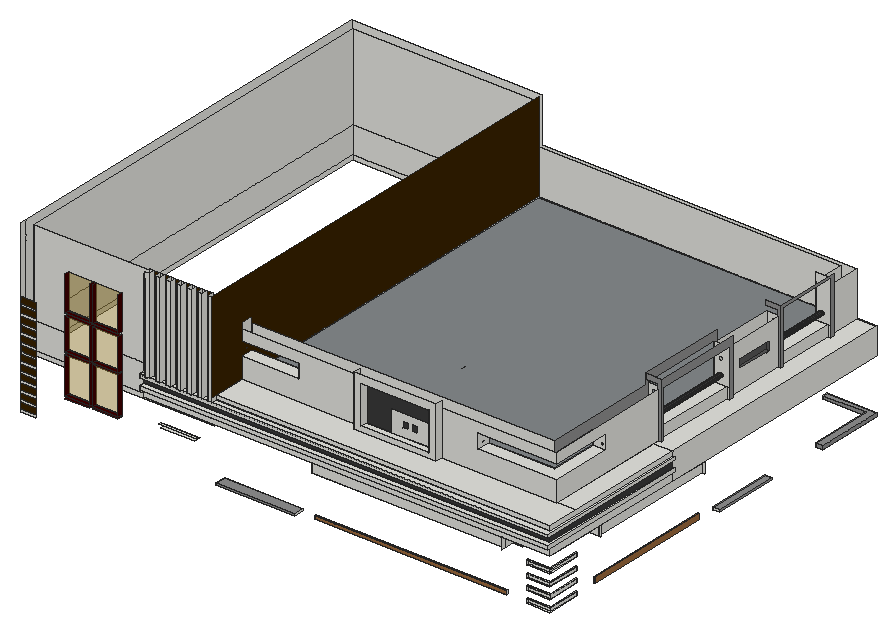
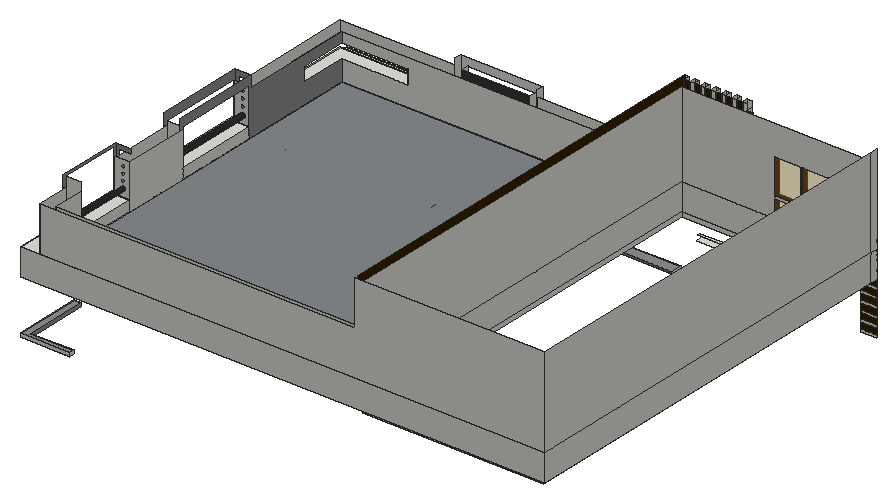
# SketchUp Ruby script. Lengths in inches.
U = 1.inch
M = Sketchup.active_model
def pt(a) = Geom::Point3d.new(a.map { |v| v * U })
def face(e, loops, mat)
  f = e.add_face(loops[0].map { |a| pt(a) })
  loops[1..].each { |l| e.add_face(l.map { |a| pt(a) }).erase! }
  f.material = f.back_material = mat if mat
  f
end
# faces: each face lists its corners as indices into pts; further lists are holes
def faces(e, pts, list, mat = nil) = list.each { |f| face(e, (f[0].is_a?(Array) ? f : [f]).map { |l| l.map { |i| pts[i] } }, mat) }
# xy, xz, yz: faces in a plane at the given z, y or x. An outline is a flat list of corners, or four numbers for a rectangle; further outlines are holes
def ring(l) = l.size == 4 ? [[l[0], l[1]], [l[2], l[1]], [l[2], l[3]], [l[0], l[3]]] : l.each_slice(2).to_a
def flat(e, list, mat, &to3) = list.each { |f| face(e, (f[0].is_a?(Array) ? f : [f]).map { |l| ring(l).map { |u, v| to3.(u, v) } }, mat) }
def xy(e, z, list, mat = nil) = flat(e, list, mat) { |x, y| [x, y, z] }
def xz(e, y, list, mat = nil) = flat(e, list, mat) { |x, z| [x, y, z] }
def yz(e, x, list, mat = nil) = flat(e, list, mat) { |y, z| [x, y, z] }
def lines(e, pts, list) = list.each { |a, b| e.add_line(pt(pts[a]), pt(pts[b])) }
# prism: a flat outline (further loops are holes) pulled along v
def prism(e, loops, v, mat = nil)
  f = face(e, loops, mat); d = Geom::Vector3d.new(v.map { |x| x * U })
  f.pushpull(f.normal.samedirection?(d) ? d.length : -d.length)
end
def box(e, o, s, mat = nil) = prism(e, [[o, [o[0] + s[0], o[1], o[2]], [o[0] + s[0], o[1] + s[1], o[2]], [o[0], o[1] + s[1], o[2]]]], [0, 0, s[2]], mat)
def at(x, y, z, deg = 0) = Geom::Transformation.translation(pt([x, y, z])) * Geom::Transformation.rotation(ORIGIN, Z_AXIS, deg.degrees)
def axes(o, x, y, z) = Geom::Transformation.new([*x, 0, *y, 0, *z, 0, *pt(o).to_a, 1])
def part(name) = M.definitions.add(name)
# library, detail: a bought-in or finely detailed component or shape, given as its bounding box
def library(name, o, s) = part(name).tap { |d| box(d.entities, o, s) }
def detail(e, o, s) = box(e.add_group.entities, o, s)
def put(e, d, t, mat = nil) = e.add_instance(d, t).tap { |i| i.material = mat if mat }
def group(e, t, mat = nil) = e.add_group.tap { |g| g.transformation = t; g.material = mat if mat }.entities
root = M.entities
M.materials.add("[Blacktop Old 01]").color = [132, 136, 139]
M.materials.add("[Color A08]").color = [56, 34, 0]
M.materials.add("[Color A08]1").color = [63, 0, 0]
M.materials.add("[Color M04]").color = [142, 142, 142]
M.materials.add("[Color M06]").color = [86, 86, 86]
M.materials.add("[Color M07]").color = [58, 58, 58]
M.materials.add("[Translucent Glass Blue]").color = [179, 149, 61]
M.materials["[Translucent Glass Blue]"].alpha = 0.5
M.materials.add("[Wood Floor]").color = [155, 105, 61]
xy(root,249,[[329.75,496.71,434.48,511.31],[455.35,504.34,712.1,506.34],[767.0625,581.49,769.0625,754.59],[767.1875,780.03,776.3125,867.13],[767.1875,951.14,767.1875,1035.15,710.3125,1035.15,710.3125,1041.15,776.3125,1041.15,776.3125,951.14]])
xy(root,249.35,[[739.88,502.4,771.75,502.4,771.75,547.34,770.25,547.34,770.25,504.84,739.88,504.84]])
xy(root,251.5625,[[329.75,496.71,434.48,511.31]],"[Color M04]")
xy(root,252.0625,[[767.1875,780.03,776.3125,867.13]],"[Color M04]")
xy(root,253.3125,[[455.35,504.34,712.1,506.34]],"[Wood Floor]")
xy(root,253.6875,[[767.1875,951.14,776.3125,951.14,776.3125,1041.15,710.3125,1041.15,710.3125,1035.15,767.1875,1035.15]],"[Color M04]")
xy(root,254.73,[[739.88,502.4,745.57,504.84],[745.57,502.4,771.75,504.84],[770.25,504.84,771.75,547.34]])
xy(root,256.0625,[[767.0625,581.49,769.0625,754.59]],"[Wood Floor]")
xy(root,264.67,[[739.88,502.4,771.75,502.4,771.75,547.34,770.25,547.34,770.25,504.77,739.88,504.77]])
xy(root,270.04,[[739.88,502.4,745.57,504.77],[745.57,502.4,771.75,504.77],[770.25,504.77,771.75,547.34]])
xy(root,279.42,[[739.88,502.4,771.75,502.4,771.75,547.34,770.0625,547.34,770.0625,504.4,739.88,504.4]])
xy(root,281.9,[[128.05,496.71,161.69,502.71],[165.04,496.71,198.99,502.71]],"[Color A08]1")
xy(root,284.79,[[739.88,502.4,745.57,504.4],[745.57,502.4,771.75,504.4],[770.0625,504.4,771.75,547.34]])
xy(root,284.92,[[128.05,496.71,161.69,502.71],[165.04,496.71,198.99,502.71]],"[Color A08]1")
xy(root,285,[[470.51,700.96,518.51,706.96]])
xy(root,286.38,[[560.85,700.96,616.42,706.96]])
xy(root,294.03,[[258.89,493.59,303.7,502.71]])
xy(root,295.73,[[739.88,502.4,745.57,504.65],[745.57,502.4,771.75,504.65],[769.8125,504.65,771.75,547.34]])
xy(root,297.5625,[[255.94,493.59,306.57,496.71]])
xy(root,301.1,[[739.88,502.4,745.57,504.65],[745.57,502.4,771.75,504.65],[769.8125,504.65,771.75,547.34]])
xy(root,306.3125,[[454.78,500.59,454.78,515.78,724.73,515.78,724.73,514.59,712.1,514.59,712.1,500.59],[758.97,581.49,758.0625,754.59,772.875,754.59,772.875,581.49]])
xy(root,321,[[329.75,496.71,329.75,700.96,710.3125,700.96,710.3125,1041.15,776.3125,1041.15,776.3125,780.03,758.0625,780.03,758.0625,754.59,758.97,581.49,758.97,566.61,724.73,566.61,724.73,515.78,455.35,515.78,455.35,516.84,434.48,516.84,434.48,496.71],[434.48,496.71,454.78,496.71,454.78,515.78,455.35,515.78,455.35,516.84,434.48,516.84],[454.78,496.71,455.35,500.59],[455.35,496.71,712.1,500.59],[712.1,496.71,724.73,514.59],
  [724.73,496.71,776.3125,502.4],[454.78,500.59,455.35,515.78],[455.35,500.59,712.1,500.59,712.1,514.59,724.73,514.59,724.73,515.78,455.35,515.78],[771.75,502.4,776.3125,566.61],[758.97,566.61,776.3125,581.49],
  [758.97,581.49,772.875,581.49,772.875,754.59,758.0625,754.59],[772.875,581.49,776.3125,700.96],[772.875,700.96,776.3125,754.59]])
xy(root,332.8125,[[233.4,489.27,776.3125,496.71],[776.3125,489.27,779.5,700.96],[329.75,496.71,776.3125,700.96]])
xy(root,334.65,[[128.05,496.71,161.69,502.71],[165.04,496.71,198.99,502.71]],"[Color A08]1")
xy(root,337.4375,[[233.4,489.27,779.5,489.27,779.5,700.96,776.3125,700.96,776.3125,496.71,233.4,496.71],[329.75,496.71,776.3125,700.96]])
xy(root,337.67,[[128.05,496.71,161.69,502.71],[165.04,496.71,198.99,502.71]],"[Color A08]1")
xy(root,347.125,[[233.4,489.27,776.3125,496.71],[776.3125,489.27,779.5,700.96],[329.75,496.71,776.3125,700.96]])
xy(root,351,[[329.75,706.96,689.4375,1035.15]])
xy(root,351.3125,[[241.19,489.02,247.4,489.27],[255.19,489.02,261.4,489.27],[269.19,489.02,275.4,489.27],[283.19,489.02,289.4,489.27],[297.19,489.02,303.4,489.27],
  [233.4,489.27,241.19,496.71],[241.19,489.27,247.4,496.71],[247.4,489.27,255.19,496.71],[255.19,489.27,261.4,496.71],[261.4,489.27,269.19,496.71],
  [269.19,489.27,275.4,496.71],[275.4,489.27,283.19,496.71],[283.19,489.27,289.4,496.71],[289.4,489.27,297.19,496.71],[297.19,489.27,303.4,496.71],
  [303.4,489.27,311.19,496.71],[311.19,489.27,317.4,496.71],[317.4,489.27,325.19,496.71],[325.19,489.27,329.75,496.71],[329.75,489.27,779.5,489.27,779.5,700.96,776.3125,700.96,776.3125,496.71,329.75,496.71]])
xy(root,357,[[329.75,496.71,776.3125,496.71,776.3125,539.27,597.14,539.27,597.14,529.59,488.01,529.59,488.01,539.27,329.75,539.27],[488.01,529.59,597.14,539.27],[329.75,539.27,750.625,539.27,750.625,700.96,733.6875,700.96,733.6875,557.27,329.75,557.27],[750.625,539.27,776.3125,700.96],[733.6875,700.96,733.6875,712.4,754.75,712.4,754.75,709.18,750.625,709.18,750.625,700.96],
  [750.625,700.96,750.625,709.18,754.75,709.18,754.75,712.4,750.625,712.4,750.625,823.78,754.75,823.78,754.75,828.03,750.625,828.03,750.625,909.39,754.75,909.39,754.75,912.34,750.625,912.34,750.625,992.73,754.75,992.73,754.75,996.8,750.625,996.8,750.625,1041.15,776.3125,1041.15,776.3125,700.96],[733.6875,823.78,733.6875,912.34,754.75,912.34,754.75,909.39,750.625,909.39,750.625,828.03,754.75,828.03,754.75,823.78]])
xy(root,357,[[329.75,557.27,733.6875,1035.15]],"[Blacktop Old 01]")
xy(root,363.72,[[496.66,529.59,587.54,539.27]])
xy(root,371.375,[[733.6875,712.4,750.625,823.78],[733.6875,912.34,750.625,992.73]])
xy(root,380.84,[[128.05,496.71,161.69,502.71],[165.04,496.71,198.99,502.71]],"[Color A08]1")
xy(root,383.25,[[746.25,843.78,750.625,894.65]],"[Color M06]")
xy(root,383.86,[[128.05,496.71,161.69,502.71],[165.04,496.71,198.99,502.71]],"[Color A08]1")
xy(root,384.48,[[329.75,539.27,405.75,557.27],[645.89,539.27,750.625,539.27,750.625,621.15,733.6875,621.15,733.6875,557.27,645.89,557.27]])
xz(root,487.84,[[75.5,251.53,96.69,254.83],[75.5,263.03,96.69,266.33],[75.5,274.53,96.69,277.83],[75.5,286.03,96.69,289.33],[75.5,297.53,96.69,300.83],
  [75.5,309.03,96.69,312.33],[75.5,320.53,96.69,323.83],[75.5,332.03,96.69,335.33],[75.5,343.53,96.69,346.83],[75.5,355.03,96.69,358.33],
  [75.5,366.53,96.69,369.83],[75.5,378.03,96.69,381.33]])
xz(root,487.84,[[75.5,254.83,96.69,263.03],[75.5,266.33,96.69,274.53],[75.5,277.83,96.69,286.03],[75.5,289.33,96.69,297.53],[75.5,300.83,96.69,309.03],
  [75.5,312.33,96.69,320.53],[75.5,323.83,96.69,332.03],[75.5,335.33,96.69,343.53],[75.5,346.83,96.69,355.03],[75.5,358.33,96.69,366.53],
  [75.5,369.83,96.69,378.03],[75.5,381.33,96.69,389.53]],"[Color A08]")
xz(root,489.02,[[241.19,351.3125,247.4,477],[255.19,351.3125,261.4,477],[269.19,351.3125,275.4,477],[283.19,351.3125,289.4,477],[297.19,351.3125,303.4,477]])
xz(root,489.27,[[233.4,332.8125,779.5,337.4375],[233.4,347.125,779.5,351.3125],[311.19,351.3125,317.4,477],[325.19,351.3125,329.75,477]])
xz(root,496.71,[[233.4,321,776.3125,332.8125],[233.4,332.8125,776.3125,337.4375],[233.4,347.125,776.3125,351.3125],[241.19,351.3125,247.4,477],[255.19,351.3125,261.4,477],
  [269.19,351.3125,275.4,477],[283.19,351.3125,289.4,477],[297.19,351.3125,303.4,477],[311.19,351.3125,317.4,477],[329.75,351.3125,776.3125,357]])
xz(root,496.71,[[233.4,351.3125,241.19,468.42],[247.4,351.3125,255.19,477],[261.4,351.3125,269.19,477],[275.4,351.3125,283.19,477],[289.4,351.3125,297.19,477],
  [303.4,351.3125,311.19,477],[317.4,351.3125,325.19,477]],"[Color A08]")
xz(root,496.71,[[329.75,249,434.48,251.5625]],"[Color M04]")
xz(root,496.71,[[233.4,337.4375,776.3125,347.125]],"[Color M07]")
xz(root,500.59,[[454.78,306.3125,712.1,321]])
xz(root,502.71,[[128.05,281.9,161.69,284.92],[161.69,281.9,165.04,284.92],[165.04,281.9,198.99,284.92],[161.69,284.92,165.04,334.65],[81.5,315,128.05,321],
  [198.99,315,323.75,321],[81.5,321,128.05,357],[198.99,321,323.75,357],[128.05,334.65,161.69,337.67],[161.69,334.65,165.04,337.67],
  [165.04,334.65,198.99,337.67],[161.69,337.67,165.04,380.84],[81.5,357,81.5,471,323.75,471,323.75,357,198.99,357,198.99,430.67,128.05,430.67,128.05,357],[128.05,380.84,161.69,383.86],[161.69,380.84,165.04,383.86],
  [165.04,380.84,198.99,383.86],[161.69,383.86,165.04,430.67]])
xz(root,502.71,[[128.05,284.92,161.69,334.65],[165.04,284.92,198.99,334.65],[128.05,337.67,161.69,380.84],[165.04,337.67,198.99,380.84],[128.05,383.86,161.69,430.67],
  [165.04,383.86,198.99,430.67]],"[Translucent Glass Blue]")
xz(root,504.34,[[455.35,249,712.1,253.3125]],"[Wood Floor]")
xz(root,504.4,[[739.88,279.42,770.0625,284.79]])
xz(root,504.65,[[739.88,295.73,769.8125,301.1]])
xz(root,504.77,[[739.88,264.67,770.25,270.04]])
xz(root,504.84,[[739.88,249.35,770.25,254.73]])
xz(root,506.34,[[455.35,249,712.1,253.3125]],"[Wood Floor]")
xz(root,511.31,[[329.75,249,434.48,251.5625]],"[Color M04]")
xz(root,514.59,[[712.1,306.3125,724.73,321]])
xz(root,515.78,[[454.78,306.3125,724.73,321]])
xz(root,529.59,[[[488.01,357,597.14,425.5625],[496.66,363.72,587.54,415.22]]])
xz(root,539.27,[[329.75,357,488.01,357,488.01,417,329.75,417,329.75,403.48,405.75,403.48,405.75,384.48,329.75,384.48],[488.01,357,488.01,384.48,496.66,384.48,496.66,363.72,587.54,363.72,587.54,384.48,597.14,384.48,597.14,357],[597.14,357,750.625,357,750.625,384.48,645.89,384.48,645.89,403.48,750.625,403.48,750.625,417,597.14,417],[[530.24,363.72,587.54,391.72],[545.17,374.78,553.48,383.09],[557.23,374.78,565.54,383.09]],[488.01,384.48,496.66,403.48],
  [587.54,384.48,597.14,403.48]])
xz(root,539.27,[[496.66,363.72,530.24,363.72,530.24,391.72,587.54,391.72,587.54,415.22,496.66,415.22],[545.17,374.78,553.48,383.09],[557.23,374.78,565.54,383.09]],"[Color M07]")
xz(root,547.34,[[770.25,249.35,771.75,254.73],[770.25,264.67,771.75,270.04],[770.0625,279.42,771.75,284.79],[769.8125,295.73,771.75,301.1]])
xz(root,557.27,[[329.75,351,733.6875,357],[329.75,357,329.75,384.48,405.75,384.48,405.75,403.48,329.75,403.48,329.75,417,733.6875,417,733.6875,403.48,645.89,403.48,645.89,384.48,733.6875,384.48,733.6875,357]])
xz(root,581.49,[[767.0625,249,769.0625,256.0625],[758.97,306.3125,772.875,321],[772.875,306.3125,776.3125,321]])
xz(root,621.15,[[[733.6875,384.48,750.625,403.48],[745.76,387.84,745.2,387.91,744.67,388.13,744.22,388.48,743.87,388.93,743.65,389.46,743.58,390.02,743.65,390.59,743.87,391.12,744.22,391.57,744.67,391.92,745.2,392.14,745.76,392.21,746.33,392.14,746.86,391.92,747.31,391.57,747.66,391.12,747.875,390.59,747.95,390.02,747.875,389.46,747.66,388.93,747.31,388.48,746.86,388.13,746.33,387.91],[741.89,395.96,741.32,396.04,740.79,396.25,740.34,396.6,739.99,397.06,739.78,397.58,739.7,398.15,739.78,398.72,739.99,399.24,740.34,399.7,740.79,400.04,741.32,400.26,741.89,400.34,742.45,400.26,742.98,400.04,743.44,399.7,743.78,399.24,744,398.72,744.08,398.15,744,397.58,743.78,397.06,743.44,396.6,742.98,396.25,742.45,396.04]]])
xz(root,700.96,[[329.75,332.8125,776.3125,337.4375],[776.3125,332.8125,779.5,337.4375],[329.75,337.4375,776.3125,347.125],[329.75,347.125,776.3125,351.3125],[776.3125,347.125,779.5,351.3125]])
xz(root,706.96,[[329.75,321,689.4375,351]])
xz(root,709.18,[[750.625,357,754.75,357,754.75,431.5625,733.6875,431.5625,733.6875,424.875,750.625,424.875]],"[Color M04]")
xz(root,712.4,[[733.6875,357,750.625,371.375],[[750.625,357,750.625,371.375,733.6875,371.375,733.6875,419.97,754.75,419.97,754.75,357],[742.21,378.95,742.97,379.05,743.68,379.34,744.29,379.81,744.75,380.42,745.05,381.125,745.15,381.89,745.05,382.65,744.75,383.36,744.29,383.96,743.68,384.43,742.97,384.72,742.21,384.82,741.45,384.72,740.74,384.43,740.13,383.96,739.67,383.36,739.37,382.65,739.27,381.89,739.37,381.125,739.67,380.42,740.13,379.81,740.74,379.34,741.45,379.05],[742.21,389.57,742.97,389.67,743.68,389.97,744.29,390.43,744.75,391.04,745.05,391.75,745.15,392.51,745.05,393.27,744.75,393.98,744.29,394.59,743.68,395.06,742.97,395.35,742.21,395.45,741.45,395.35,740.74,395.06,740.13,394.59,739.67,393.98,739.37,393.27,739.27,392.51,739.37,391.75,739.67,391.04,740.13,390.43,740.74,389.97,741.45,389.67],[742.21,399.14,742.97,399.24,743.68,399.53,744.29,400,744.75,400.61,745.05,401.3125,745.15,402.07,745.05,402.83,744.75,403.54,744.29,404.15,743.68,404.62,742.97,404.91,742.21,405.01,741.45,404.91,740.74,404.62,740.13,404.15,739.67,403.54,739.37,402.83,739.27,402.07,739.37,401.3125,739.67,400.61,740.13,400,740.74,399.53,741.45,399.24],[742.21,408.57,742.97,408.67,743.68,408.97,744.29,409.43,744.75,410.04,745.05,410.75,745.15,411.51,745.05,412.27,744.75,412.98,744.29,413.59,743.68,414.06,742.97,414.35,742.21,414.45,741.45,414.35,740.74,414.06,740.13,413.59,739.67,412.98,739.37,412.27,739.27,411.51,739.37,410.75,739.67,410.04,740.13,409.43,740.74,408.97,741.45,408.67]],[742.21,378.95,742.97,379.05,743.68,379.34,744.29,379.81,744.75,380.42,745.05,381.125,745.15,381.89,745.05,382.65,744.75,383.36,744.29,383.96,743.68,384.43,742.97,384.72,742.21,384.82,741.45,384.72,740.74,384.43,740.13,383.96,739.67,383.36,739.37,382.65,739.27,381.89,739.37,381.125,739.67,380.42,740.13,379.81,740.74,379.34,741.45,379.05]])
xz(root,754.59,[[767.0625,249,769.0625,256.0625],[758.0625,306.3125,772.875,321],[772.875,306.3125,776.3125,321]])
xz(root,780.03,[[767.1875,249,776.3125,252.0625]])
xz(root,823.78,[[733.6875,357,750.625,371.375],[750.625,357,754.75,371.375],[[733.6875,371.375,754.75,419.97],[742.21,399.14,741.45,399.24,740.74,399.53,740.13,400,739.67,400.61,739.37,401.3125,739.27,402.07,739.37,402.83,739.67,403.54,740.13,404.15,740.74,404.62,741.45,404.91,742.21,405.01,742.97,404.91,743.68,404.62,744.29,404.15,744.75,403.54,745.05,402.83,745.15,402.07,745.05,401.3125,744.75,400.61,744.29,400,743.68,399.53,742.97,399.24]]])
xz(root,824.72,[[742.21,378.95,741.45,379.05,740.74,379.34,740.13,379.81,739.67,380.42,739.37,381.125,739.27,381.89,739.37,382.65,739.67,383.36,740.13,383.96,740.74,384.43,741.45,384.72,742.21,384.82,742.97,384.72,743.68,384.43,744.29,383.96,744.75,383.36,745.05,382.65,745.15,381.89,745.05,381.125,744.75,380.42,744.29,379.81,743.68,379.34,742.97,379.05]])
xz(root,828.03,[[750.625,357,754.75,417]],"[Color M04]")
xz(root,843.78,[[746.25,383.25,750.625,396]],"[Color M06]")
xz(root,867.13,[[767.1875,249,776.3125,252.0625]],"[Color M04]")
xz(root,894.65,[[746.25,383.25,750.625,396]],"[Color M06]")
xz(root,909.39,[[750.625,357,754.75,357,754.75,431.5625,733.6875,431.5625,733.6875,424.875,750.625,424.875]],"[Color M04]")
xz(root,912.34,[[733.6875,357,750.625,371.375],[750.625,357,754.75,371.375],[[733.6875,371.375,754.75,417],[741.96,379.46,742.64,379.55,743.28,379.81,743.82,380.23,744.24,380.77,744.5,381.4,744.59,382.08,744.5,382.76,744.24,383.4,743.82,383.9375,743.28,384.36,742.64,384.62,741.96,384.71,741.28,384.62,740.65,384.36,740.11,383.9375,739.69,383.4,739.43,382.76,739.34,382.08,739.43,381.4,739.69,380.77,740.11,380.23,740.65,379.81,741.28,379.55],[741.96,388.71,742.64,388.8,743.28,389.06,743.82,389.48,744.24,390.02,744.5,390.65,744.59,391.33,744.5,392.01,744.24,392.65,743.82,393.1875,743.28,393.61,742.64,393.87,741.96,393.96,741.28,393.87,740.65,393.61,740.11,393.1875,739.69,392.65,739.43,392.01,739.34,391.33,739.43,390.65,739.69,390.02,740.11,389.48,740.65,389.06,741.28,388.8],[741.96,397.33,742.64,397.42,743.28,397.68,743.82,398.1,744.24,398.65,744.5,399.28,744.59,399.96,744.5,400.64,744.24,401.27,743.82,401.8125,743.28,402.23,742.64,402.49,741.96,402.58,741.28,402.49,740.65,402.23,740.11,401.8125,739.69,401.27,739.43,400.64,739.34,399.96,739.43,399.28,739.69,398.65,740.11,398.1,740.65,397.68,741.28,397.42],[741.96,406.27,742.64,406.36,743.28,406.62,743.82,407.04,744.24,407.58,744.5,408.22,744.59,408.9,744.5,409.57,744.24,410.21,743.82,410.75,743.28,411.17,742.64,411.43,741.96,411.52,741.28,411.43,740.65,411.17,740.11,410.75,739.69,410.21,739.43,409.57,739.34,408.9,739.43,408.22,739.69,407.58,740.11,407.04,740.65,406.62,741.28,406.36]],[741.96,379.46,742.64,379.55,743.28,379.81,743.82,380.23,744.24,380.77,744.5,381.4,744.59,382.08,744.5,382.76,744.24,383.4,743.82,383.9375,743.28,384.36,742.64,384.62,741.96,384.71,741.28,384.62,740.65,384.36,740.11,383.9375,739.69,383.4,739.43,382.76,739.34,382.08,739.43,381.4,739.69,380.77,740.11,380.23,740.65,379.81,741.28,379.55]])
xz(root,951.14,[[767.1875,249,776.3125,253.6875]],"[Color M04]")
xz(root,992.73,[[733.6875,357,750.625,371.375],[750.625,357,754.75,371.375],[733.6875,371.375,754.75,428.02]])
xz(root,992.84,[[741.96,379.46,741.28,379.55,740.65,379.81,740.11,380.23,739.69,380.77,739.43,381.4,739.34,382.08,739.43,382.76,739.69,383.4,740.11,383.9375,740.65,384.36,741.28,384.62,741.96,384.71,742.64,384.62,743.28,384.36,743.82,383.9375,744.24,383.4,744.5,382.76,744.59,382.08,744.5,381.4,744.24,380.77,743.82,380.23,743.28,379.81,742.64,379.55]])
xz(root,996.8,[[750.625,357,754.75,417]],"[Color M04]")
xz(root,1035.15,[[81.5,315,323.75,321],[81.5,321,323.75,357],[329.75,321,689.4375,351],[329.75,351,689.4375,357],[689.4375,351,733.6875,357],
  [81.5,357,323.75,471],[329.75,357,733.6875,417]])
xz(root,1035.15,[[710.3125,249,767.1875,253.6875]],"[Color M04]")
xz(root,1041.15,[[710.3125,249,776.3125,253.6875],[75.5,321,776.3125,357],[75.5,357,75.5,477,329.75,477,329.75,417,750.625,417,750.625,357]])
yz(root,75.5,[[487.84,321,496.71,357],[496.71,321,1041.15,357],[487.84,357,496.71,477],[496.71,357,1041.15,477]])
yz(root,81.5,[[502.71,315,1035.15,321],[502.71,321,1035.15,357],[502.71,357,1035.15,471]])
yz(root,128.05,[[496.71,284.92,502.71,334.65],[496.71,337.67,502.71,380.84],[496.71,383.86,502.71,430.67]],"[Color A08]1")
yz(root,161.69,[[496.71,284.92,502.71,334.65],[496.71,337.67,502.71,380.84],[496.71,383.86,502.71,430.67]],"[Color A08]1")
yz(root,165.04,[[496.71,284.92,502.71,334.65],[496.71,337.67,502.71,380.84],[496.71,383.86,502.71,430.67]],"[Color A08]1")
yz(root,198.99,[[496.71,284.92,502.71,334.65],[496.71,337.67,502.71,380.84],[496.71,383.86,502.71,430.67]],"[Color A08]1")
yz(root,233.4,[[489.27,332.8125,496.71,337.4375],[489.27,347.125,496.71,351.3125]])
yz(root,241.19,[[489.02,351.3125,496.71,468.42]])
yz(root,247.4,[[489.02,351.3125,496.71,477]])
yz(root,255.19,[[489.02,351.3125,496.71,477]])
yz(root,261.4,[[489.02,351.3125,496.71,477]])
yz(root,269.19,[[489.02,351.3125,496.71,477]])
yz(root,275.4,[[489.02,351.3125,496.71,477]])
yz(root,283.19,[[489.02,351.3125,496.71,477]])
yz(root,289.4,[[489.02,351.3125,496.71,477]])
yz(root,297.19,[[489.02,351.3125,496.71,477]])
yz(root,303.4,[[489.02,351.3125,496.71,477]])
yz(root,311.19,[[489.27,351.3125,496.71,477]])
yz(root,317.4,[[489.27,351.3125,496.71,477]])
yz(root,323.75,[[502.71,315,1035.15,321],[502.71,321,1035.15,357],[502.71,357,1035.15,471]])
yz(root,325.19,[[489.27,351.3125,496.71,477]])
yz(root,329.75,[[496.71,249,511.31,251.5625],[706.96,321,1035.15,351],[557.27,351,700.96,351.3125],[700.96,351,706.96,357],[706.96,351,1035.15,357],
  [489.27,351.3125,496.71,357],[496.71,351.3125,557.27,357],[557.27,351.3125,700.96,357]])
yz(root,329.75,[[[489.27,357,539.27,357,539.27,384.48,557.27,384.48,557.27,403.48,539.27,403.48,539.27,424.875,557.27,424.875,557.27,357,1035.15,357,1035.15,477,489.27,477],[548.47,388.74,547.92,388.81,547.41,389.02,546.97,389.36,546.63,389.8,546.42,390.3125,546.35,390.86,546.42,391.41,546.63,391.92,546.97,392.36,547.41,392.7,547.92,392.91,548.47,392.99,549.02,392.91,549.53,392.7,549.97,392.36,550.3125,391.92,550.52,391.41,550.6,390.86,550.52,390.3125,550.3125,389.8,549.97,389.36,549.53,389.02,549.02,388.81],[548.47,397.42,547.92,397.5,547.41,397.71,546.97,398.05,546.63,398.49,546.42,399,546.35,399.55,546.42,400.1,546.63,400.61,546.97,401.05,547.41,401.39,547.92,401.6,548.47,401.67,549.02,401.6,549.53,401.39,549.97,401.05,550.3125,400.61,550.52,400.1,550.6,399.55,550.52,399,550.3125,398.49,549.97,398.05,549.53,397.71,549.02,397.5]]],"[Color A08]")
yz(root,405.75,[[[539.27,384.48,557.27,403.48],[548.47,388.74,549.02,388.81,549.53,389.02,549.97,389.36,550.3125,389.8,550.52,390.3125,550.6,390.86,550.52,391.41,550.3125,391.92,549.97,392.36,549.53,392.7,549.02,392.91,548.47,392.99,547.92,392.91,547.41,392.7,546.97,392.36,546.63,391.92,546.42,391.41,546.35,390.86,546.42,390.3125,546.63,389.8,546.97,389.36,547.41,389.02,547.92,388.81],[548.47,397.42,549.02,397.5,549.53,397.71,549.97,398.05,550.3125,398.49,550.52,399,550.6,399.55,550.52,400.1,550.3125,400.61,549.97,401.05,549.53,401.39,549.02,401.6,548.47,401.67,547.92,401.6,547.41,401.39,546.97,401.05,546.63,400.61,546.42,400.1,546.35,399.55,546.42,399,546.63,398.49,546.97,398.05,547.41,397.71,547.92,397.5]]])
yz(root,434.48,[[496.71,249,511.31,251.5625]])
yz(root,454.78,[[500.59,306.3125,515.78,321]])
yz(root,455.35,[[504.34,249,506.34,253.3125]])
yz(root,488.01,[[529.59,357,539.27,425.5625]])
yz(root,496.66,[[529.59,363.72,539.27,415.22]])
yz(root,587.54,[[529.59,363.72,539.27,415.22]])
yz(root,597.14,[[529.59,357,539.27,425.5625]])
yz(root,645.89,[[[539.27,384.48,557.27,403.48],[548.01,387.84,547.45,387.91,546.92,388.13,546.47,388.48,546.12,388.93,545.9,389.46,545.83,390.02,545.9,390.59,546.12,391.12,546.47,391.57,546.92,391.92,547.45,392.14,548.01,392.21,548.58,392.14,549.11,391.92,549.5625,391.57,549.91,391.12,550.13,390.59,550.2,390.02,550.13,389.46,549.91,388.93,549.5625,388.48,549.11,388.13,548.58,387.91],[548.01,395.96,547.45,396.04,546.92,396.25,546.47,396.6,546.12,397.06,545.9,397.58,545.83,398.15,545.9,398.72,546.12,399.24,546.47,399.7,546.92,400.04,547.45,400.26,548.01,400.34,548.58,400.26,549.11,400.04,549.5625,399.7,549.91,399.24,550.13,398.72,550.2,398.15,550.13,397.58,549.91,397.06,549.5625,396.6,549.11,396.25,548.58,396.04]]])
yz(root,689.4375,[[706.96,321,1035.15,351]])
yz(root,710.3125,[[1035.15,249,1041.15,253.6875]])
yz(root,712.1,[[504.34,249,506.34,253.3125],[496.71,306.3125,500.59,321],[500.59,306.3125,514.59,321]])
yz(root,724.73,[[514.59,306.3125,515.78,321]])
yz(root,733.6875,[[557.27,351,700.96,357],[700.96,351,1035.15,357],[712.4,357,823.78,371.375],[823.78,357,912.34,417],[912.34,357,992.73,371.375],
  [992.73,357,1035.15,417]])
yz(root,733.6875,[[557.27,357,557.27,384.48,621.15,384.48,621.15,403.48,557.27,403.48,557.27,417,709.18,417,709.18,431.5625,828.03,431.5625,828.03,417,823.78,417,823.78,419.97,712.4,419.97,712.4,357]],"[Color M04]")
yz(root,739.88,[[502.4,249.35,504.84,254.73],[502.4,264.67,504.77,270.04],[502.4,279.42,504.4,284.79],[502.4,295.73,504.65,301.1]])
yz(root,746.25,[[843.78,383.25,894.65,396]],"[Color M06]")
yz(root,750.625,[[539.27,357,709.18,357,709.18,417,539.27,417,539.27,403.48,621.15,403.48,621.15,384.48,539.27,384.48],[712.4,357,823.78,371.375],[[828.03,357,909.39,417],[843.78,383.25,894.65,396]],[912.34,357,992.73,371.375],[996.8,357,1041.15,417]])
yz(root,754.75,[[709.18,357,712.4,357,712.4,419.97,823.78,419.97,823.78,357,828.03,357,828.03,431.5625,709.18,431.5625],[909.39,357,912.34,357,912.34,428.02,992.73,428.02,992.73,357,996.8,357,996.8,431.5625,909.39,431.5625]],"[Color M04]")
yz(root,767.0625,[[581.49,249,754.59,256.0625]],"[Wood Floor]")
yz(root,767.1875,[[780.03,249,867.13,252.0625],[951.14,249,1035.15,253.6875]],"[Color M04]")
yz(root,769.0625,[[581.49,249,754.59,256.0625]],"[Wood Floor]")
yz(root,769.8125,[[504.65,295.73,547.34,301.1]])
yz(root,770.0625,[[504.4,279.42,547.34,284.79]])
yz(root,770.25,[[504.84,249.35,547.34,254.73],[504.77,264.67,547.34,270.04]])
yz(root,772.875,[[581.49,306.3125,754.59,321]])
yz(root,776.3125,[[496.71,321,700.96,332.8125],[700.96,321,1041.15,357],[496.71,351.3125,700.96,357]])
yz(root,776.3125,[[780.03,249,867.13,252.0625],[951.14,249,1041.15,253.6875]],"[Color M04]")
yz(root,776.3125,[[496.71,337.4375,700.96,347.125]],"[Color M07]")
yz(root,779.5,[[489.27,332.8125,700.96,337.4375],[489.27,347.125,700.96,351.3125]])
p = [[758.97,581.49,321],[758.0625,754.59,321],[758.0625,754.59,306.3125],[758.97,581.49,306.3125],[742.21,712.4,378.95],[741.45,712.4,379.05],
  [741.45,824.72,379.05],[742.21,824.72,378.95],[742.97,712.4,379.05],[742.97,824.72,379.05],[740.74,712.4,379.34],[740.74,824.72,379.34],
  [743.68,712.4,379.34],[743.68,824.72,379.34],[740.13,712.4,379.81],[740.13,824.72,379.81],[744.29,712.4,379.81],[744.29,824.72,379.81],
  [741.28,912.34,379.55],[740.65,912.34,379.81],[740.65,992.84,379.81],[741.28,992.84,379.55],[741.96,912.34,379.46],[741.96,992.84,379.46],
  [742.64,912.34,379.55],[742.64,992.84,379.55],[743.28,912.34,379.81],[743.28,992.84,379.81],[739.67,712.4,380.42],[739.67,824.72,380.42],
  [744.75,712.4,380.42],[744.75,824.72,380.42],[740.11,912.34,380.23],[740.11,992.84,380.23],[743.82,912.34,380.23],[743.82,992.84,380.23],
  [739.69,912.34,380.77],[739.69,992.84,380.77],[744.24,912.34,380.77],[744.24,992.84,380.77],[739.37,712.4,381.125],[739.37,824.72,381.125],
  [745.05,712.4,381.125],[745.05,824.72,381.125],[739.43,912.34,381.4],[739.43,992.84,381.4],[744.5,912.34,381.4],[744.5,992.84,381.4],
  [739.27,712.4,381.89],[739.27,824.72,381.89],[745.15,712.4,381.89],[745.15,824.72,381.89],[739.34,912.34,382.08],[739.34,992.84,382.08],
  [744.59,912.34,382.08],[744.59,992.84,382.08],[739.37,712.4,382.65],[739.37,824.72,382.65],[745.05,712.4,382.65],[745.05,824.72,382.65],
  [739.43,912.34,382.76],[739.43,992.84,382.76],[744.5,912.34,382.76],[744.5,992.84,382.76],[739.67,712.4,383.36],[739.67,824.72,383.36],
  [744.75,712.4,383.36],[744.75,824.72,383.36],[739.69,912.34,383.4],[739.69,992.84,383.4],[744.24,912.34,383.4],[744.24,992.84,383.4],
  [740.13,712.4,383.96],[740.13,824.72,383.96],[744.29,712.4,383.96],[744.29,824.72,383.96],[740.11,912.34,383.9375],[740.11,992.84,383.9375],
  [743.82,912.34,383.9375],[743.82,992.84,383.9375],[740.65,912.34,384.36],[740.65,992.84,384.36],[743.28,912.34,384.36],[743.28,992.84,384.36],
  [740.74,712.4,384.43],[740.74,824.72,384.43],[743.68,712.4,384.43],[743.68,824.72,384.43],[741.45,712.4,384.72],[741.45,824.72,384.72],
  [742.97,712.4,384.72],[742.97,824.72,384.72],[741.28,912.34,384.62],[741.28,992.84,384.62],[742.64,912.34,384.62],[742.64,992.84,384.62],
  [741.96,912.34,384.71],[741.96,992.84,384.71],[742.21,712.4,384.82],[742.21,824.72,384.82],[329.75,700.96,321],[329.75,700.96,332.8125],
  [724.73,526.78,321],[728.4375,526.78,321],[494.64,706.96,357],[494.64,706.96,351],[689.4375,706.96,351],[689.4375,706.96,357],
  [494.64,700.96,357]]
faces(root,p,[[0,1,2,3]])
faces(root,p,[[4,5,6,7],[8,4,7,9],[5,10,11,6],[12,8,9,13],[10,14,15,11],[16,12,13,17],[18,19,20,21],[22,18,21,23],
  [24,22,23,25],[26,24,25,27],[14,28,29,15],[30,16,17,31],[19,32,33,20],[34,26,27,35],[32,36,37,33],[38,34,35,39],
  [28,40,41,29],[42,30,31,43],[36,44,45,37],[46,38,39,47],[40,48,49,41],[50,42,43,51],[44,52,53,45],[54,46,47,55],
  [48,56,57,49],[58,50,51,59],[52,60,61,53],[62,54,55,63],[56,64,65,57],[66,58,59,67],[60,68,69,61],[70,62,63,71],
  [64,72,73,65],[74,66,67,75],[68,76,77,69],[78,70,71,79],[76,80,81,77],[82,78,79,83],[72,84,85,73],[86,74,75,87],
  [84,88,89,85],[90,86,87,91],[80,92,93,81],[94,82,83,95],[92,96,97,93],[96,94,95,97],[88,98,99,89],[98,90,91,99]],"[Color M07]")
lines(root,p,[[100,101],[102,103],[104,105],[106,107],[104,108]])
